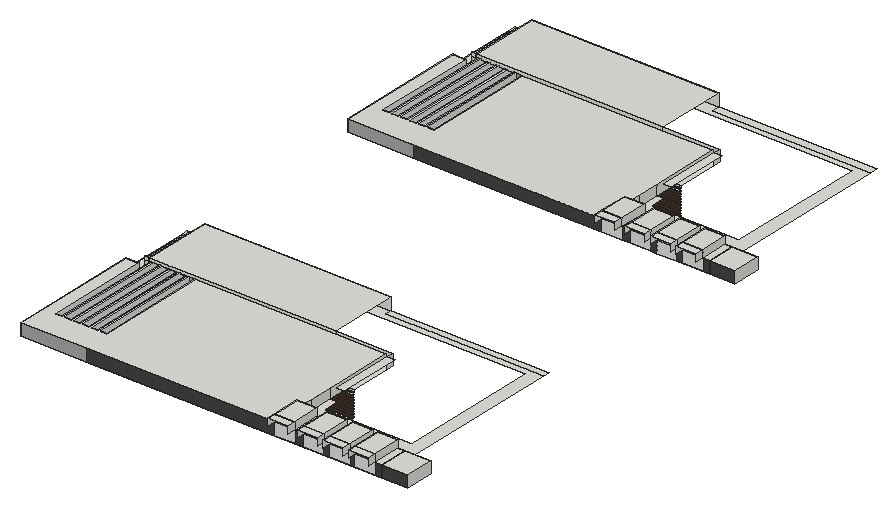
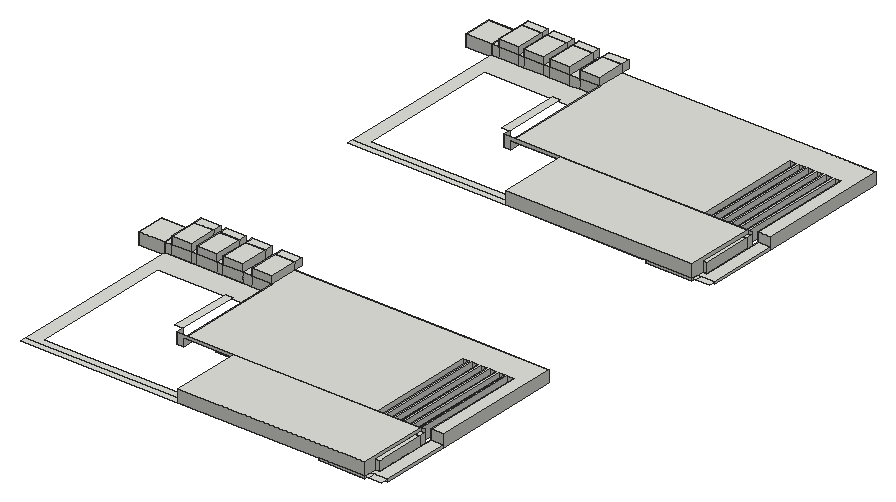
# SketchUp Ruby script. Lengths in inches.
U = 1.inch
M = Sketchup.active_model
def pt(a) = Geom::Point3d.new(a.map { |v| v * U })
def face(e, loops, mat)
  f = e.add_face(loops[0].map { |a| pt(a) })
  loops[1..].each { |l| e.add_face(l.map { |a| pt(a) }).erase! }
  f.material = f.back_material = mat if mat
  f
end
# faces: each face lists its corners as indices into pts; further lists are holes
def faces(e, pts, list, mat = nil) = list.each { |f| face(e, (f[0].is_a?(Array) ? f : [f]).map { |l| l.map { |i| pts[i] } }, mat) }
# xy, xz, yz: faces in a plane at the given z, y or x. An outline is a flat list of corners, or four numbers for a rectangle; further outlines are holes
def ring(l) = l.size == 4 ? [[l[0], l[1]], [l[2], l[1]], [l[2], l[3]], [l[0], l[3]]] : l.each_slice(2).to_a
def flat(e, list, mat, &to3) = list.each { |f| face(e, (f[0].is_a?(Array) ? f : [f]).map { |l| ring(l).map { |u, v| to3.(u, v) } }, mat) }
def xy(e, z, list, mat = nil) = flat(e, list, mat) { |x, y| [x, y, z] }
def xz(e, y, list, mat = nil) = flat(e, list, mat) { |x, z| [x, y, z] }
def yz(e, x, list, mat = nil) = flat(e, list, mat) { |y, z| [x, y, z] }
def lines(e, pts, list) = list.each { |a, b| e.add_line(pt(pts[a]), pt(pts[b])) }
# prism: a flat outline (further loops are holes) pulled along v
def prism(e, loops, v, mat = nil)
  f = face(e, loops, mat); d = Geom::Vector3d.new(v.map { |x| x * U })
  f.pushpull(f.normal.samedirection?(d) ? d.length : -d.length)
end
def box(e, o, s, mat = nil) = prism(e, [[o, [o[0] + s[0], o[1], o[2]], [o[0] + s[0], o[1] + s[1], o[2]], [o[0], o[1] + s[1], o[2]]]], [0, 0, s[2]], mat)
def at(x, y, z, deg = 0) = Geom::Transformation.translation(pt([x, y, z])) * Geom::Transformation.rotation(ORIGIN, Z_AXIS, deg.degrees)
def axes(o, x, y, z) = Geom::Transformation.new([*x, 0, *y, 0, *z, 0, *pt(o).to_a, 1])
def part(name) = M.definitions.add(name)
# library, detail: a bought-in or finely detailed component or shape, given as its bounding box
def library(name, o, s) = part(name).tap { |d| box(d.entities, o, s) }
def detail(e, o, s) = box(e.add_group.entities, o, s)
def put(e, d, t, mat = nil) = e.add_instance(d, t).tap { |i| i.material = mat if mat }
def group(e, t, mat = nil) = e.add_group.tap { |g| g.transformation = t; g.material = mat if mat }.entities
root = M.entities
M.materials.add("[Color M03]1").color = [170, 170, 170]
M.materials.add("[Color M05]").color = [68, 68, 68]
M.materials.add("[Granite Dark Gray]").color = [69, 68, 68]
M.materials.add("[Wood Veneer 01]").color = [96, 56, 29]
c1 = library("A$C06767DEF\#1",[-8.3,1.21,0],[7.09,7.09,5.51])
xy(root,437.47,[[1582.55,466.33,1669.17,468.64]])
xy(root,437.84,[[1582.21,1125.42,1668.82,1127.73]])
xy(root,438.5,[[1582.55,466.33,1669.17,468.64]])
xy(root,438.875,[[1582.21,1125.42,1668.82,1127.73]])
xy(root,441.53,[[1582.55,466.33,1669.17,468.64]])
xy(root,441.91,[[1582.21,1125.42,1668.82,1127.73]])
xy(root,442.5625,[[1582.55,466.33,1669.17,468.64]])
xy(root,442.9375,[[1582.21,1125.42,1668.82,1127.73]])
xy(root,445.59,[[1582.55,466.33,1669.17,468.64]])
xy(root,445.97,[[1582.21,1125.42,1668.82,1127.73]])
xy(root,446.625,[[1582.55,466.33,1669.17,468.64]])
xy(root,447,[[1582.21,1125.42,1668.82,1127.73]])
xy(root,449.66,[[1582.55,466.33,1669.17,468.64]])
xy(root,450.03,[[1582.21,1125.42,1668.82,1127.73]])
xy(root,450.6875,[[1582.55,466.33,1669.17,468.64]])
xy(root,451.0625,[[1582.21,1125.42,1668.82,1127.73]])
xy(root,453.72,[[1582.55,466.33,1669.17,468.64]])
xy(root,454.09,[[1582.21,1125.42,1668.82,1127.73]])
xy(root,454.75,[[1582.55,466.33,1669.17,468.64]])
xy(root,455.125,[[1582.21,1125.42,1668.82,1127.73]])
xy(root,457.78,[[1582.55,466.33,1669.17,468.64]])
xy(root,458.16,[[1582.21,1125.42,1668.82,1127.73]])
xy(root,458.8125,[[1582.55,466.33,1669.17,468.64]])
xy(root,459.1875,[[1582.21,1125.42,1668.82,1127.73]])
xy(root,461.84,[[1582.55,466.33,1669.17,468.64]])
xy(root,462.22,[[1582.21,1125.42,1668.82,1127.73]])
xy(root,462.875,[[1582.55,466.33,1669.17,468.64]])
xy(root,463.25,[[1582.21,1125.42,1668.82,1127.73]])
xy(root,465.91,[[1582.55,466.33,1669.17,468.64]])
xy(root,466.28,[[1582.21,1125.42,1668.82,1127.73]])
xy(root,466.9375,[[1582.55,466.33,1669.17,468.64]])
xy(root,467.3125,[[1582.21,1125.42,1668.82,1127.73]])
xy(root,469.97,[[1582.55,466.33,1669.17,468.64]])
xy(root,470.34,[[1582.21,1125.42,1668.82,1127.73]])
xy(root,471,[[1582.55,466.33,1669.17,468.64]])
xy(root,471.375,[[1582.21,1125.42,1668.82,1127.73]])
xy(root,471.94,[[1831.09,322.97,1872.84,368.59],[1582.55,466.33,1657.65,468.64],[1276.37,647.98,1350.61,659.09]])
xy(root,471.94,[[[1248.34,322.97,1248.34,647.98,1269.46,647.98,1269.46,546.92,1269.17,546.92,1269.17,368.83,1279.04,368.83,1279.04,556.89,1276.37,556.89,1276.37,557.39,1269.46,557.39,1269.46,637.97,1276.37,637.97,1276.37,647.98,1350.61,647.98,1350.61,546.92,1340.73,546.92,1340.73,368.83,1350.61,368.83,1350.61,340.27,1353.51,322.97],[1326.42,368.83,1336.29,557.39],[1312.11,368.83,1321.98,557.39],[1297.79,368.83,1307.67,557.39],[1283.48,368.83,1293.36,557.39]]],"[Color M03]1")
xy(root,471.94,[[1353.51,322.97,1350.61,340.27,1831.09,340.27,1831.09,322.97]],"[Color M05]")
xy(root,474.03,[[1657.65,466.33,1669.17,468.64]])
xy(root,474.41,[[1582.21,1125.42,1668.82,1127.73]])
xy(root,475.4375,[[1582.21,1125.42,1668.82,1127.73]])
xy(root,475.57,[[1350.61,340.27,1350.61,637.97,1356.97,637.97,1356.97,534.98,1582.55,534.98,1582.55,466.33,1657.65,466.33,1657.65,368.59,1831.09,368.59,1831.09,340.27],[1657.65,368.59,1831.09,368.59,1831.09,647.98,1576.68,647.98,1576.68,659.09,1356.97,659.09,1356.97,637.97,1809.97,637.97,1809.97,408.96,1669.17,408.96,1669.17,433.78,1657.65,433.78],[1248.34,534.98,1269.17,534.98,1269.17,546.92,1269.46,546.92,1269.46,637.97,1350.61,637.97,1350.61,647.98,1248.34,647.98],[1350.61,637.97,1356.97,647.98],[1248.34,647.98,1269.46,659.09],
  [1269.46,647.98,1276.37,659.09],[1276.37,647.98,1350.61,659.09],[1350.61,647.98,1356.97,659.09],[1576.68,647.98,1831.09,659.09]])
xy(root,476.38,[[1830.75,982.06,1872.5,1027.68],[1582.21,1125.42,1657.31,1127.73],[1276.02,1307.07,1350.26,1318.18]])
xy(root,476.38,[[[1248,982.06,1248,1307.07,1269.12,1307.07,1269.12,1206.01,1268.82,1206.01,1268.82,1027.92,1278.7,1027.92,1278.7,1215.98,1276.02,1215.98,1276.02,1216.48,1269.12,1216.48,1269.12,1297.06,1276.02,1297.06,1276.02,1307.07,1350.26,1307.07,1350.26,1206.01,1340.39,1206.01,1340.39,1027.92,1350.26,1027.92,1350.26,999.36,1353.16,982.06],[1326.07,1027.92,1335.95,1216.48],[1311.76,1027.92,1321.64,1216.48],[1297.45,1027.92,1307.32,1216.48],[1283.14,1027.92,1293.01,1216.48]]],"[Color M03]1")
xy(root,476.38,[[1353.16,982.06,1350.26,999.36,1830.75,999.36,1830.75,982.06]],"[Color M05]")
xy(root,478.09,[[1657.65,468.64,1669.17,546.92]])
xy(root,478.47,[[1657.31,1125.42,1668.82,1127.73]])
xy(root,480,[[1350.26,999.36,1350.26,1297.06,1356.62,1297.06,1356.62,1194.07,1582.21,1194.07,1582.21,1125.42,1657.31,1125.42,1657.31,1027.68,1830.75,1027.68,1830.75,999.36],[1657.31,1027.68,1830.75,1027.68,1830.75,1307.07,1576.34,1307.07,1576.34,1318.18,1356.62,1318.18,1356.62,1297.06,1809.63,1297.06,1809.63,1068.05,1668.82,1068.05,1668.82,1092.87,1657.31,1092.87],[1248,1194.07,1268.82,1194.07,1268.82,1206.01,1269.12,1206.01,1269.12,1297.06,1350.26,1297.06,1350.26,1307.07,1248,1307.07],[1350.26,1297.06,1356.62,1307.07],[1248,1307.07,1269.12,1318.18],
  [1269.12,1307.07,1276.02,1318.18],[1276.02,1307.07,1350.26,1318.18],[1350.26,1307.07,1356.62,1318.18],[1576.34,1307.07,1830.75,1318.18]])
xy(root,482.53,[[1657.31,1127.73,1668.82,1206.01]])
xy(root,491.07,[[1248.34,322.97,1657.65,322.97,1657.65,546.92,1350.61,546.92,1350.61,368.83,1340.73,368.83,1340.73,546.92,1336.29,546.92,1336.29,368.83,1326.42,368.83,1326.42,546.92,1321.98,546.92,1321.98,368.83,1312.11,368.83,1312.11,546.92,1307.67,546.92,1307.67,368.83,1297.79,368.83,1297.79,546.92,1293.36,546.92,1293.36,368.83,1283.48,368.83,1283.48,546.92,1279.04,546.92,1279.04,368.83,1269.17,368.83,1269.17,534.98,1248.34,534.98],[1657.65,322.97,1689.86,368.59],[1689.86,322.97,1705.34,368.59],[1705.34,322.97,1737.55,368.59],[1737.55,322.97,1746.96,368.59],
  [1746.96,322.97,1779.17,368.59],[1779.17,322.97,1787.59,368.59],[1787.59,322.97,1819.8,368.59],[1819.8,322.97,1831.09,368.59],[1831.09,322.97,1872.84,368.59],
  [1269.46,546.92,1276.37,557.39],[1276.37,546.92,1279.04,556.89],[1283.48,546.92,1293.36,557.39],[1297.79,546.92,1307.67,557.39],[1312.11,546.92,1321.98,557.39],
  [1326.42,546.92,1336.29,557.39],[1276.37,556.89,1279.04,572.79],[1269.46,557.39,1276.37,637.97]])
xy(root,495.5,[[1248,982.06,1657.31,982.06,1657.31,1206.01,1350.26,1206.01,1350.26,1027.92,1340.39,1027.92,1340.39,1206.01,1335.95,1206.01,1335.95,1027.92,1326.07,1027.92,1326.07,1206.01,1321.64,1206.01,1321.64,1027.92,1311.76,1027.92,1311.76,1206.01,1307.32,1206.01,1307.32,1027.92,1297.45,1027.92,1297.45,1206.01,1293.01,1206.01,1293.01,1027.92,1283.14,1027.92,1283.14,1206.01,1278.7,1206.01,1278.7,1027.92,1268.82,1027.92,1268.82,1194.07,1248,1194.07],[1657.31,982.06,1689.52,1027.68],[1689.52,982.06,1705,1027.68],[1705,982.06,1737.2,1027.68],[1737.2,982.06,1746.62,1027.68],
  [1746.62,982.06,1778.83,1027.68],[1778.83,982.06,1787.25,1027.68],[1787.25,982.06,1819.45,1027.68],[1819.45,982.06,1830.75,1027.68],[1830.75,982.06,1872.5,1027.68],
  [1269.12,1206.01,1276.02,1216.48],[1276.02,1206.01,1278.7,1215.98],[1283.14,1206.01,1293.01,1216.48],[1297.45,1206.01,1307.32,1216.48],[1311.76,1206.01,1321.64,1216.48],
  [1326.07,1206.01,1335.95,1216.48],[1276.02,1215.98,1278.7,1231.88],[1269.12,1216.48,1276.02,1297.06]])
xy(root,496.07,[[1669.17,433.78,1681.11,534.98],[1276.37,546.92,1576.68,659.09]])
xy(root,500.5,[[1668.82,1092.87,1680.76,1194.07],[1276.02,1206.01,1576.34,1318.18]])
xy(root,502.82,[[1657.65,309.65,1689.86,322.97],[1705.34,309.65,1737.55,322.97],[1746.96,309.65,1779.17,322.97],[1787.59,309.65,1819.8,322.97],[1657.65,322.97,1689.86,368.59],
  [1705.34,322.97,1737.55,368.59],[1746.96,322.97,1779.17,368.59],[1787.59,322.97,1819.8,368.59]])
xy(root,507.25,[[1657.31,968.74,1689.52,982.06],[1705,968.74,1737.2,982.06],[1746.62,968.74,1778.83,982.06],[1787.25,968.74,1819.45,982.06],[1657.31,982.06,1689.52,1027.68],
  [1705,982.06,1737.2,1027.68],[1746.62,982.06,1778.83,1027.68],[1787.25,982.06,1819.45,1027.68]])
xz(root,322.97,[[1657.65,471.94,1689.86,491.07],[1705.34,471.94,1737.55,491.07],[1746.96,471.94,1779.17,491.07],[1787.59,471.94,1819.8,491.07],[1657.65,491.07,1689.86,502.82],
  [1705.34,491.07,1737.55,502.82],[1746.96,491.07,1779.17,502.82],[1787.59,491.07,1819.8,502.82]])
xz(root,322.97,[[1248.34,471.94,1353.51,491.07]],"[Color M03]1")
xz(root,322.97,[[1353.51,471.94,1657.65,491.07],[1689.86,471.94,1705.34,491.07],[1737.55,471.94,1746.96,491.07],[1779.17,471.94,1787.59,491.07],[1819.8,471.94,1831.09,491.07],
  [1831.09,471.94,1872.84,491.07]],"[Granite Dark Gray]")
xz(root,340.27,[[1350.61,471.94,1831.09,475.57]])
xz(root,368.59,[[1831.09,471.94,1872.84,491.07],[1657.65,475.57,1689.86,491.07],[1689.86,475.57,1705.34,491.07],[1705.34,475.57,1737.55,491.07],[1737.55,475.57,1746.96,491.07],
  [1746.96,475.57,1779.17,491.07],[1779.17,475.57,1787.59,491.07],[1787.59,475.57,1819.8,491.07],[1819.8,475.57,1831.09,491.07],[1657.65,491.07,1689.86,502.82],
  [1705.34,491.07,1737.55,502.82],[1746.96,491.07,1779.17,502.82],[1787.59,491.07,1819.8,502.82]])
xz(root,368.83,[[1269.17,471.94,1279.04,491.07],[1283.48,471.94,1293.36,491.07],[1297.79,471.94,1307.67,491.07],[1312.11,471.94,1321.98,491.07],[1326.42,471.94,1336.29,491.07],
  [1340.73,471.94,1350.61,491.07]])
xz(root,466.33,[[1582.55,471,1669.17,471,1669.17,474.03,1657.65,474.03,1657.65,471.94,1582.55,471.94]])
xz(root,466.33,[[1582.55,438.5,1669.17,441.53],[1582.55,442.5625,1669.17,445.59],[1582.55,446.625,1669.17,449.66],[1582.55,450.6875,1669.17,453.72],[1582.55,454.75,1669.17,457.78],
  [1582.55,458.8125,1669.17,461.84],[1582.55,462.875,1669.17,465.91],[1582.55,466.9375,1669.17,469.97],[1582.55,471.94,1657.65,475.57]],"[Wood Veneer 01]")
xz(root,468.64,[[1582.55,437.47,1669.17,438.5],[1582.55,441.53,1669.17,442.5625],[1582.55,445.59,1669.17,446.625],[1582.55,449.66,1669.17,450.6875],[1582.55,453.72,1669.17,454.75],
  [1582.55,457.78,1669.17,458.8125],[1582.55,461.84,1669.17,462.875],[1582.55,465.91,1669.17,466.9375],[1582.55,469.97,1669.17,471],[1582.55,471.94,1657.65,474.03],
  [1657.65,474.03,1669.17,475.0625],[1582.55,475.0625,1657.65,478.09],[1657.65,475.0625,1669.17,478.09]])
xz(root,534.98,[[1248.34,475.57,1269.17,491.07]])
xz(root,546.92,[[1269.17,471.94,1269.46,475.57],[1657.65,478.09,1657.65,491.07,1576.68,491.07,1576.68,496.07,1669.17,496.07,1669.17,478.09],[1269.46,491.07,1276.37,496.07],[1276.37,491.07,1576.68,496.07]])
xz(root,546.92,[[1340.73,471.94,1350.61,491.07]],"[Color M03]1")
xz(root,556.89,[[1276.37,471.94,1279.04,491.07]])
xz(root,557.39,[[1269.46,471.82,1276.37,471.94]])
xz(root,557.39,[[1269.46,471.94,1276.37,491.07],[1283.48,471.94,1293.36,491.07],[1297.79,471.94,1307.67,491.07],[1312.11,471.94,1321.98,491.07],[1326.42,471.94,1336.29,491.07]],"[Color M03]1")
xz(root,637.97,[[1269.46,471.82,1276.37,471.94],[1269.46,471.94,1276.37,475.57],[1269.46,475.57,1276.37,491.07]])
xz(root,647.98,[[1276.37,471.94,1350.61,475.57]])
xz(root,659.09,[[1276.37,471.94,1350.61,475.57],[1276.37,475.57,1576.68,496.07]])
xz(root,982.06,[[1657.31,476.38,1689.52,495.5],[1705,476.38,1737.2,495.5],[1746.62,476.38,1778.83,495.5],[1787.25,476.38,1819.45,495.5],[1657.31,495.5,1689.52,507.25],
  [1705,495.5,1737.2,507.25],[1746.62,495.5,1778.83,507.25],[1787.25,495.5,1819.45,507.25]])
xz(root,982.06,[[1248,476.38,1353.16,495.5]],"[Color M03]1")
xz(root,982.06,[[1353.16,476.38,1657.31,495.5],[1689.52,476.38,1705,495.5],[1737.2,476.38,1746.62,495.5],[1778.83,476.38,1787.25,495.5],[1819.45,476.38,1830.75,495.5],
  [1830.75,476.38,1872.5,495.5]],"[Granite Dark Gray]")
xz(root,999.36,[[1350.26,476.38,1830.75,480]])
xz(root,1027.68,[[1830.75,476.38,1872.5,495.5],[1657.31,480,1689.52,495.5],[1689.52,480,1705,495.5],[1705,480,1737.2,495.5],[1737.2,480,1746.62,495.5],
  [1746.62,480,1778.83,495.5],[1778.83,480,1787.25,495.5],[1787.25,480,1819.45,495.5],[1819.45,480,1830.75,495.5],[1657.31,495.5,1689.52,507.25],
  [1705,495.5,1737.2,507.25],[1746.62,495.5,1778.83,507.25],[1787.25,495.5,1819.45,507.25]])
xz(root,1027.92,[[1268.82,476.38,1278.7,495.5],[1283.14,476.38,1293.01,495.5],[1297.45,476.38,1307.32,495.5],[1311.76,476.38,1321.64,495.5],[1326.07,476.38,1335.95,495.5],
  [1340.39,476.38,1350.26,495.5]])
xz(root,1125.42,[[1582.21,475.4375,1668.82,475.4375,1668.82,478.47,1657.31,478.47,1657.31,476.38,1582.21,476.38]])
xz(root,1125.42,[[1582.21,438.875,1668.82,441.91],[1582.21,442.9375,1668.82,445.97],[1582.21,447,1668.82,450.03],[1582.21,451.0625,1668.82,454.09],[1582.21,455.125,1668.82,458.16],
  [1582.21,459.1875,1668.82,462.22],[1582.21,463.25,1668.82,466.28],[1582.21,467.3125,1668.82,470.34],[1582.21,471.375,1668.82,474.41],[1582.21,476.38,1657.31,480]],"[Wood Veneer 01]")
xz(root,1127.73,[[1582.21,437.84,1668.82,438.875],[1582.21,441.91,1668.82,442.9375],[1582.21,445.97,1668.82,447],[1582.21,450.03,1668.82,451.0625],[1582.21,454.09,1668.82,455.125],
  [1582.21,458.16,1668.82,459.1875],[1582.21,462.22,1668.82,463.25],[1582.21,466.28,1668.82,467.3125],[1582.21,470.34,1668.82,471.375],[1582.21,474.41,1668.82,475.4375],
  [1582.21,476.38,1657.31,478.47],[1657.31,478.47,1668.82,479.5],[1582.21,479.5,1657.31,482.53],[1657.31,479.5,1668.82,482.53]])
xz(root,1194.07,[[1248,480,1268.82,495.5]])
xz(root,1206.01,[[1268.82,476.38,1269.12,480],[1657.31,482.53,1657.31,495.5,1576.34,495.5,1576.34,500.5,1668.82,500.5,1668.82,482.53],[1269.12,495.5,1276.02,500.5],[1276.02,495.5,1576.34,500.5]])
xz(root,1206.01,[[1340.39,476.38,1350.26,495.5]],"[Color M03]1")
xz(root,1215.98,[[1276.02,476.38,1278.7,495.5]])
xz(root,1216.48,[[1269.12,476.25,1276.02,476.38]])
xz(root,1216.48,[[1269.12,476.38,1276.02,495.5],[1283.14,476.38,1293.01,495.5],[1297.45,476.38,1307.32,495.5],[1311.76,476.38,1321.64,495.5],[1326.07,476.38,1335.95,495.5]],"[Color M03]1")
xz(root,1297.06,[[1269.12,476.25,1276.02,476.38],[1269.12,476.38,1276.02,480],[1269.12,480,1276.02,495.5]])
xz(root,1307.07,[[1276.02,476.38,1350.26,480]])
xz(root,1318.18,[[1276.02,476.38,1350.26,480],[1276.02,480,1576.34,500.5]])
yz(root,1248,[[982.06,476.38,1194.07,495.5],[1194.07,476.38,1307.07,480]])
yz(root,1248.34,[[322.97,471.94,534.98,491.07],[534.98,471.94,647.98,475.57]])
yz(root,1268.82,[[1027.92,476.38,1206.01,476.38,1206.01,480,1194.07,480,1194.07,495.5,1027.92,495.5]])
yz(root,1269.12,[[1216.48,476.25,1297.06,476.38],[1206.01,476.38,1216.48,480],[1216.48,476.38,1297.06,480],[1206.01,480,1216.48,495.5],[1216.48,480,1297.06,495.5]])
yz(root,1269.17,[[368.83,471.94,546.92,471.94,546.92,475.57,534.98,475.57,534.98,491.07,368.83,491.07]])
yz(root,1269.46,[[557.39,471.82,637.97,471.94],[546.92,471.94,557.39,475.57],[557.39,471.94,637.97,475.57],[546.92,475.57,557.39,491.07],[557.39,475.57,637.97,491.07]])
yz(root,1276.02,[[1297.06,476.38,1297.06,495.5,1206.01,495.5,1206.01,500.5,1318.18,500.5,1318.18,480,1307.07,480,1307.07,476.38],[1215.98,476.38,1216.48,495.5],[1307.07,476.38,1318.18,480]])
yz(root,1276.37,[[637.97,471.94,637.97,491.07,546.92,491.07,546.92,496.07,659.09,496.07,659.09,475.57,647.98,475.57,647.98,471.94],[556.89,471.94,557.39,491.07],[647.98,471.94,659.09,475.57]])
yz(root,1278.7,[[1027.92,476.38,1215.98,495.5]])
yz(root,1279.04,[[368.83,471.94,556.89,491.07]])
yz(root,1283.14,[[1027.92,476.38,1216.48,495.5]])
yz(root,1283.48,[[368.83,471.94,557.39,491.07]])
yz(root,1293.01,[[1027.92,476.38,1216.48,495.5]])
yz(root,1293.36,[[368.83,471.94,557.39,491.07]])
yz(root,1297.45,[[1027.92,476.38,1216.48,495.5]])
yz(root,1297.79,[[368.83,471.94,557.39,491.07]])
yz(root,1307.32,[[1027.92,476.38,1216.48,495.5]])
yz(root,1307.67,[[368.83,471.94,557.39,491.07]])
yz(root,1311.76,[[1027.92,476.38,1216.48,495.5]])
yz(root,1312.11,[[368.83,471.94,557.39,491.07]])
yz(root,1321.64,[[1027.92,476.38,1216.48,495.5]])
yz(root,1321.98,[[368.83,471.94,557.39,491.07]])
yz(root,1326.07,[[1027.92,476.38,1216.48,495.5]])
yz(root,1326.42,[[368.83,471.94,557.39,491.07]])
yz(root,1335.95,[[1027.92,476.38,1216.48,495.5]])
yz(root,1336.29,[[368.83,471.94,557.39,491.07]])
yz(root,1340.39,[[1027.92,476.38,1206.01,495.5]])
yz(root,1340.73,[[368.83,471.94,546.92,491.07]])
yz(root,1350.26,[[999.36,476.38,1027.92,480],[1206.01,476.38,1307.07,480],[1307.07,476.38,1318.18,480],[1027.92,480,1206.01,495.5]])
yz(root,1350.61,[[340.27,471.94,368.83,475.57],[546.92,471.94,647.98,475.57],[647.98,471.94,659.09,475.57],[368.83,475.57,546.92,491.07]])
yz(root,1582.21,[[1125.42,476.38,1127.73,480]])
yz(root,1582.55,[[466.33,471.94,468.64,475.57]])
yz(root,1657.31,[[1125.42,476.38,1127.73,478.47],[1125.42,478.47,1127.73,478.47,1127.73,482.53,1206.01,482.53,1206.01,495.5,1092.87,495.5,1092.87,480,1125.42,480],[1027.68,480,1056.54,495.5],[1056.54,480,1092.87,495.5],[968.74,495.5,982.06,507.25],
  [982.06,495.5,1027.68,507.25]])
yz(root,1657.65,[[466.33,471.94,468.64,474.03],[466.33,474.03,468.64,474.03,468.64,478.09,546.92,478.09,546.92,491.07,433.78,491.07,433.78,475.57,466.33,475.57],[368.59,475.57,397.45,491.07],[397.45,475.57,433.78,491.07],[309.65,491.07,322.97,502.82],
  [322.97,491.07,368.59,502.82]])
yz(root,1668.82,[[1194.07,482.53,1206.01,500.5]])
yz(root,1669.17,[[534.98,478.09,546.92,496.07]])
yz(root,1689.52,[[968.74,495.5,982.06,507.25],[982.06,495.5,1027.68,507.25]])
yz(root,1689.86,[[309.65,491.07,322.97,502.82],[322.97,491.07,368.59,502.82]])
yz(root,1705,[[968.74,495.5,982.06,507.25],[982.06,495.5,1027.68,507.25]])
yz(root,1705.34,[[309.65,491.07,322.97,502.82],[322.97,491.07,368.59,502.82]])
yz(root,1737.2,[[968.74,495.5,982.06,507.25],[982.06,495.5,1027.68,507.25]])
yz(root,1737.55,[[309.65,491.07,322.97,502.82],[322.97,491.07,368.59,502.82]])
yz(root,1746.62,[[968.74,495.5,982.06,507.25],[982.06,495.5,1027.68,507.25]])
yz(root,1746.96,[[309.65,491.07,322.97,502.82],[322.97,491.07,368.59,502.82]])
yz(root,1778.83,[[968.74,495.5,982.06,507.25],[982.06,495.5,1027.68,507.25]])
yz(root,1779.17,[[309.65,491.07,322.97,502.82],[322.97,491.07,368.59,502.82]])
yz(root,1787.25,[[968.74,495.5,982.06,507.25],[982.06,495.5,1027.68,507.25]])
yz(root,1787.59,[[309.65,491.07,322.97,502.82],[322.97,491.07,368.59,502.82]])
yz(root,1819.45,[[968.74,495.5,982.06,507.25],[982.06,495.5,1027.68,507.25]])
yz(root,1819.8,[[309.65,491.07,322.97,502.82],[322.97,491.07,368.59,502.82]])
yz(root,1830.75,[[982.06,476.38,999.36,476.38,999.36,480,1027.68,480,1027.68,495.5,982.06,495.5],[999.36,476.38,1027.68,480]])
yz(root,1831.09,[[322.97,471.94,340.27,471.94,340.27,475.57,368.59,475.57,368.59,491.07,322.97,491.07],[340.27,471.94,368.59,475.57]])
yz(root,1872.5,[[982.06,476.38,1027.68,495.5]])
yz(root,1872.84,[[322.97,471.94,368.59,491.07]])
put(root,c1,at(1389.18,1092.87,474.49))
put(root,c1,at(1389.52,433.78,470.05))
put(root,c1,at(1463.8,1092.87,474.49))
put(root,c1,at(1464.15,433.78,470.05))
put(root,c1,at(1541.99,1092.87,474.49))
put(root,c1,at(1542.33,433.78,470.05))
